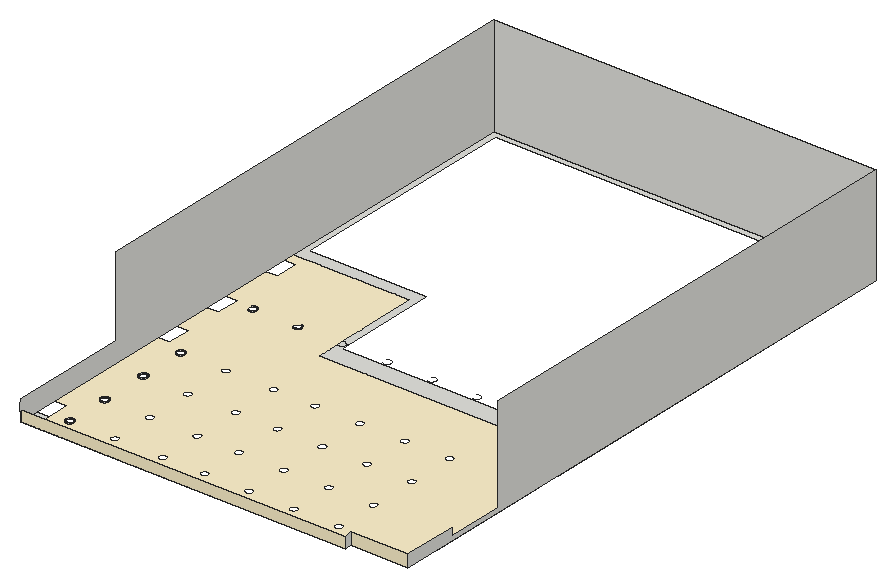
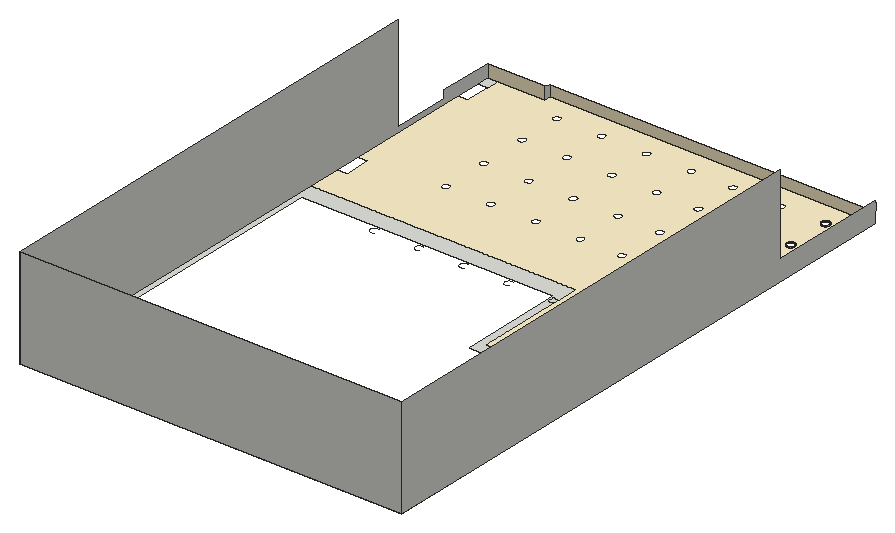
# SketchUp Ruby script. Lengths in inches.
U = 1.inch
M = Sketchup.active_model
def pt(a) = Geom::Point3d.new(a.map { |v| v * U })
def face(e, loops, mat)
  f = e.add_face(loops[0].map { |a| pt(a) })
  loops[1..].each { |l| e.add_face(l.map { |a| pt(a) }).erase! }
  f.material = f.back_material = mat if mat
  f
end
# faces: each face lists its corners as indices into pts; further lists are holes
def faces(e, pts, list, mat = nil) = list.each { |f| face(e, (f[0].is_a?(Array) ? f : [f]).map { |l| l.map { |i| pts[i] } }, mat) }
# xy, xz, yz: faces in a plane at the given z, y or x. An outline is a flat list of corners, or four numbers for a rectangle; further outlines are holes
def ring(l) = l.size == 4 ? [[l[0], l[1]], [l[2], l[1]], [l[2], l[3]], [l[0], l[3]]] : l.each_slice(2).to_a
def flat(e, list, mat, &to3) = list.each { |f| face(e, (f[0].is_a?(Array) ? f : [f]).map { |l| ring(l).map { |u, v| to3.(u, v) } }, mat) }
def xy(e, z, list, mat = nil) = flat(e, list, mat) { |x, y| [x, y, z] }
def xz(e, y, list, mat = nil) = flat(e, list, mat) { |x, z| [x, y, z] }
def yz(e, x, list, mat = nil) = flat(e, list, mat) { |y, z| [x, y, z] }
def lines(e, pts, list) = list.each { |a, b| e.add_line(pt(pts[a]), pt(pts[b])) }
# prism: a flat outline (further loops are holes) pulled along v
def prism(e, loops, v, mat = nil)
  f = face(e, loops, mat); d = Geom::Vector3d.new(v.map { |x| x * U })
  f.pushpull(f.normal.samedirection?(d) ? d.length : -d.length)
end
def box(e, o, s, mat = nil) = prism(e, [[o, [o[0] + s[0], o[1], o[2]], [o[0] + s[0], o[1] + s[1], o[2]], [o[0], o[1] + s[1], o[2]]]], [0, 0, s[2]], mat)
def at(x, y, z, deg = 0) = Geom::Transformation.translation(pt([x, y, z])) * Geom::Transformation.rotation(ORIGIN, Z_AXIS, deg.degrees)
def axes(o, x, y, z) = Geom::Transformation.new([*x, 0, *y, 0, *z, 0, *pt(o).to_a, 1])
def part(name) = M.definitions.add(name)
# library, detail: a bought-in or finely detailed component or shape, given as its bounding box
def library(name, o, s) = part(name).tap { |d| box(d.entities, o, s) }
def detail(e, o, s) = box(e.add_group.entities, o, s)
def put(e, d, t, mat = nil) = e.add_instance(d, t).tap { |i| i.material = mat if mat }
def group(e, t, mat = nil) = e.add_group.tap { |g| g.transformation = t; g.material = mat if mat }.entities
root = M.entities
M.materials.add("[Color D01]").color = [255, 242, 204]
xy(root,126,[[177.75,359.375,193.125,383.3125],[644.75,368.125,657.75,383.3125],[[324.13,645.5,324.13,673.57,324.96,672.9375,326.17,672.4375,327.46,672.27,328.76,672.4375,329.96,672.9375,331,673.73,331.79,674.77,332.29,675.97,332.46,677.27,332.29,678.5625,331.79,679.77,331,680.8,329.96,681.6,328.76,682.1,327.46,682.27,326.17,682.1,324.96,681.6,324.13,680.96,324.13,788.13,177.75,788.13,177.75,1103.3125,657.75,1103.3125,657.75,645.5],[332.57,669.6875,650.24,669.6875,650.24,1095.81,185.26,1095.81,185.26,802.9375,332.57,802.9375]],[327.46,672.27,326.17,672.4375,324.96,672.9375,324.13,673.57,324.13,680.96,324.96,681.6,326.17,682.1,327.46,682.27,328.76,682.1,329.96,681.6,331,680.8,331.79,679.77,332.29,678.5625,332.46,677.27,332.29,675.97,331.79,674.77,331,673.73,329.96,672.9375,328.76,672.4375]])
xy(root,126,[[[193.125,359.375,193.125,412.64,177.75,412.64,177.75,575.25,192.5,575.25,192.5,604.58,177.75,604.58,177.75,651.6,192.5,651.6,192.5,680.93,177.75,680.93,177.75,744.25,192.5,744.25,192.5,773.58,177.75,773.58,177.75,788.13,324.13,788.13,324.13,645.5,657.75,645.5,657.75,604.54,644.75,604.54,644.75,572.73,657.75,572.73,657.75,415.125,644.75,415.125,644.75,368.125,585.62,368.125,585.62,359.375],[271.15,500.05,272.44,500.22,273.65,500.72,274.68,501.52,275.48,502.55,275.98,503.76,276.15,505.05,275.98,506.35,275.48,507.55,274.68,508.59,273.65,509.38,272.44,509.88,271.15,510.05,269.86,509.88,268.65,509.38,267.61,508.59,266.82,507.55,266.32,506.35,266.15,505.05,266.32,503.76,266.82,502.55,267.61,501.52,268.65,500.72,269.86,500.22],[440.09,500.05,441.38,500.22,442.59,500.72,443.62,501.52,444.42,502.55,444.92,503.76,445.09,505.05,444.92,506.35,444.42,507.55,443.62,508.59,442.59,509.38,441.38,509.88,440.09,510.05,438.79,509.88,437.59,509.38,436.55,508.59,435.76,507.55,435.26,506.35,435.09,505.05,435.26,503.76,435.76,502.55,436.55,501.52,437.59,500.72,438.79,500.22],[496.4,500.05,497.69,500.22,498.9,500.72,499.93,501.52,500.73,502.55,501.23,503.76,501.4,505.05,501.23,506.35,500.73,507.55,499.93,508.59,498.9,509.38,497.69,509.88,496.4,510.05,495.11,509.88,493.9,509.38,492.86,508.59,492.07,507.55,491.57,506.35,491.4,505.05,491.57,503.76,492.07,502.55,492.86,501.52,493.9,500.72,495.11,500.22],[552.71,500.05,554.01,500.22,555.21,500.72,556.25,501.52,557.04,502.55,557.54,503.76,557.71,505.05,557.54,506.35,557.04,507.55,556.25,508.59,555.21,509.38,554.01,509.88,552.71,510.05,551.42,509.88,550.21,509.38,549.18,508.59,548.38,507.55,547.88,506.35,547.71,505.05,547.88,503.76,548.38,502.55,549.18,501.52,550.21,500.72,551.42,500.22],[271.15,439.5625,272.44,439.73,273.65,440.23,274.68,441.03,275.48,442.0625,275.98,443.27,276.15,444.5625,275.98,445.86,275.48,447.0625,274.68,448.1,273.65,448.89,272.44,449.39,271.15,449.5625,269.86,449.39,268.65,448.89,267.61,448.1,266.82,447.0625,266.32,445.86,266.15,444.5625,266.32,443.27,266.82,442.0625,267.61,441.03,268.65,440.23,269.86,439.73],[440.09,439.5625,441.38,439.73,442.59,440.23,443.62,441.03,444.42,442.0625,444.92,443.27,445.09,444.5625,444.92,445.86,444.42,447.0625,443.62,448.1,442.59,448.89,441.38,449.39,440.09,449.5625,438.79,449.39,437.59,448.89,436.55,448.1,435.76,447.0625,435.26,445.86,435.09,444.5625,435.26,443.27,435.76,442.0625,436.55,441.03,437.59,440.23,438.79,439.73],[496.4,439.5625,497.69,439.73,498.9,440.23,499.93,441.03,500.73,442.0625,501.23,443.27,501.4,444.5625,501.23,445.86,500.73,447.0625,499.93,448.1,498.9,448.89,497.69,449.39,496.4,449.5625,495.11,449.39,493.9,448.89,492.86,448.1,492.07,447.0625,491.57,445.86,491.4,444.5625,491.57,443.27,492.07,442.0625,492.86,441.03,493.9,440.23,495.11,439.73],[552.71,439.5625,554.01,439.73,555.21,440.23,556.25,441.03,557.04,442.0625,557.54,443.27,557.71,444.5625,557.54,445.86,557.04,447.0625,556.25,448.1,555.21,448.89,554.01,449.39,552.71,449.5625,551.42,449.39,550.21,448.89,549.18,448.1,548.38,447.0625,547.88,445.86,547.71,444.5625,547.88,443.27,548.38,442.0625,549.18,441.03,550.21,440.23,551.42,439.73],[271.15,672.27,272.44,672.4375,273.65,672.9375,274.68,673.73,275.48,674.77,275.98,675.97,276.15,677.27,275.98,678.5625,275.48,679.77,274.68,680.8,273.65,681.6,272.44,682.1,271.15,682.27,269.86,682.1,268.65,681.6,267.61,680.8,266.82,679.77,266.32,678.5625,266.15,677.27,266.32,675.97,266.82,674.77,267.61,673.73,268.65,672.9375,269.86,672.4375],[271.15,559.33,272.44,559.5,273.65,560,274.68,560.79,275.48,561.83,275.98,563.03,276.15,564.33,275.98,565.62,275.48,566.83,274.68,567.86,273.65,568.66,272.44,569.16,271.15,569.33,269.86,569.16,268.65,568.66,267.61,567.86,266.82,566.83,266.32,565.62,266.15,564.33,266.32,563.03,266.82,561.83,267.61,560.79,268.65,560,269.86,559.5],[440.09,559.33,441.38,559.5,442.59,560,443.62,560.79,444.42,561.83,444.92,563.03,445.09,564.33,444.92,565.62,444.42,566.83,443.62,567.86,442.59,568.66,441.38,569.16,440.09,569.33,438.79,569.16,437.59,568.66,436.55,567.86,435.76,566.83,435.26,565.62,435.09,564.33,435.26,563.03,435.76,561.83,436.55,560.79,437.59,560,438.79,559.5],[496.4,559.33,497.69,559.5,498.9,560,499.93,560.79,500.73,561.83,501.23,563.03,501.4,564.33,501.23,565.62,500.73,566.83,499.93,567.86,498.9,568.66,497.69,569.16,496.4,569.33,495.11,569.16,493.9,568.66,492.86,567.86,492.07,566.83,491.57,565.62,491.4,564.33,491.57,563.03,492.07,561.83,492.86,560.79,493.9,560,495.11,559.5],[552.71,559.33,554.01,559.5,555.21,560,556.25,560.79,557.04,561.83,557.54,563.03,557.71,564.33,557.54,565.62,557.04,566.83,556.25,567.86,555.21,568.66,554.01,569.16,552.71,569.33,551.42,569.16,550.21,568.66,549.18,567.86,548.38,566.83,547.88,565.62,547.71,564.33,547.88,563.03,548.38,561.83,549.18,560.79,550.21,560,551.42,559.5],[271.15,385.12,272.44,385.29,273.65,385.79,274.68,386.58,275.48,387.62,275.98,388.83,276.15,390.12,275.98,391.41,275.48,392.62,274.68,393.66,273.65,394.45,272.44,394.95,271.15,395.12,269.86,394.95,268.65,394.45,267.61,393.66,266.82,392.62,266.32,391.41,266.15,390.12,266.32,388.83,266.82,387.62,267.61,386.58,268.65,385.79,269.86,385.29],[440.09,385.12,441.38,385.29,442.59,385.79,443.62,386.58,444.42,387.62,444.92,388.83,445.09,390.12,444.92,391.41,444.42,392.62,443.62,393.66,442.59,394.45,441.38,394.95,440.09,395.12,438.79,394.95,437.59,394.45,436.55,393.66,435.76,392.62,435.26,391.41,435.09,390.12,435.26,388.83,435.76,387.62,436.55,386.58,437.59,385.79,438.79,385.29],[496.4,385.12,497.69,385.29,498.9,385.79,499.93,386.58,500.73,387.62,501.23,388.83,501.4,390.12,501.23,391.41,500.73,392.62,499.93,393.66,498.9,394.45,497.69,394.95,496.4,395.12,495.11,394.95,493.9,394.45,492.86,393.66,492.07,392.62,491.57,391.41,491.4,390.12,491.57,388.83,492.07,387.62,492.86,386.58,493.9,385.79,495.11,385.29],[552.71,385.12,554.01,385.29,555.21,385.79,556.25,386.58,557.04,387.62,557.54,388.83,557.71,390.12,557.54,391.41,557.04,392.62,556.25,393.66,555.21,394.45,554.01,394.95,552.71,395.12,551.42,394.95,550.21,394.45,549.18,393.66,548.38,392.62,547.88,391.41,547.71,390.12,547.88,388.83,548.38,387.62,549.18,386.58,550.21,385.79,551.42,385.29],[214.84,672.27,216.13,672.4375,217.34,672.9375,218.37,673.73,219.17,674.77,219.67,675.97,219.84,677.27,219.67,678.5625,219.17,679.77,218.37,680.8,217.34,681.6,216.13,682.1,214.84,682.27,213.54,682.1,212.34,681.6,211.3,680.8,210.51,679.77,210.01,678.5625,209.84,677.27,210.01,675.97,210.51,674.77,211.3,673.73,212.34,672.9375,213.54,672.4375],[214.84,439.5625,216.13,439.73,217.34,440.23,218.37,441.03,219.17,442.0625,219.67,443.27,219.84,444.5625,219.67,445.86,219.17,447.0625,218.37,448.1,217.34,448.89,216.13,449.39,214.84,449.5625,213.54,449.39,212.34,448.89,211.3,448.1,210.51,447.0625,210.01,445.86,209.84,444.5625,210.01,443.27,210.51,442.0625,211.3,441.03,212.34,440.23,213.54,439.73],[214.84,500.05,216.13,500.22,217.34,500.72,218.37,501.52,219.17,502.55,219.67,503.76,219.84,505.05,219.67,506.35,219.17,507.55,218.37,508.59,217.34,509.38,216.13,509.88,214.84,510.05,213.54,509.88,212.34,509.38,211.3,508.59,210.51,507.55,210.01,506.35,209.84,505.05,210.01,503.76,210.51,502.55,211.3,501.52,212.34,500.72,213.54,500.22],[214.84,559.33,216.13,559.5,217.34,560,218.37,560.79,219.17,561.83,219.67,563.03,219.84,564.33,219.67,565.62,219.17,566.83,218.37,567.86,217.34,568.66,216.13,569.16,214.84,569.33,213.54,569.16,212.34,568.66,211.3,567.86,210.51,566.83,210.01,565.62,209.84,564.33,210.01,563.03,210.51,561.83,211.3,560.79,212.34,560,213.54,559.5],[214.84,385.12,216.13,385.29,217.34,385.79,218.37,386.58,219.17,387.62,219.67,388.83,219.84,390.12,219.67,391.41,219.17,392.62,218.37,393.66,217.34,394.45,216.13,394.95,214.84,395.12,213.54,394.95,212.34,394.45,211.3,393.66,210.51,392.62,210.01,391.41,209.84,390.12,210.01,388.83,210.51,387.62,211.3,386.58,212.34,385.79,213.54,385.29],[331.21,439.5625,332.51,439.73,333.71,440.23,334.75,441.03,335.54,442.0625,336.04,443.27,336.21,444.5625,336.04,445.86,335.54,447.0625,334.75,448.1,333.71,448.89,332.51,449.39,331.21,449.5625,329.92,449.39,328.71,448.89,327.68,448.1,326.88,447.0625,326.38,445.86,326.21,444.5625,326.38,443.27,326.88,442.0625,327.68,441.03,328.71,440.23,329.92,439.73],[383.77,439.5625,385.07,439.73,386.27,440.23,387.31,441.03,388.1,442.0625,388.6,443.27,388.77,444.5625,388.6,445.86,388.1,447.0625,387.31,448.1,386.27,448.89,385.07,449.39,383.77,449.5625,382.48,449.39,381.27,448.89,380.24,448.1,379.44,447.0625,378.94,445.86,378.77,444.5625,378.94,443.27,379.44,442.0625,380.24,441.03,381.27,440.23,382.48,439.73],[383.77,500.05,385.07,500.22,386.27,500.72,387.31,501.52,388.1,502.55,388.6,503.76,388.77,505.05,388.6,506.35,388.1,507.55,387.31,508.59,386.27,509.38,385.07,509.88,383.77,510.05,382.48,509.88,381.27,509.38,380.24,508.59,379.44,507.55,378.94,506.35,378.77,505.05,378.94,503.76,379.44,502.55,380.24,501.52,381.27,500.72,382.48,500.22],[331.21,500.05,332.51,500.22,333.71,500.72,334.75,501.52,335.54,502.55,336.04,503.76,336.21,505.05,336.04,506.35,335.54,507.55,334.75,508.59,333.71,509.38,332.51,509.88,331.21,510.05,329.92,509.88,328.71,509.38,327.68,508.59,326.88,507.55,326.38,506.35,326.21,505.05,326.38,503.76,326.88,502.55,327.68,501.52,328.71,500.72,329.92,500.22],[383.77,559.33,385.07,559.5,386.27,560,387.31,560.79,388.1,561.83,388.6,563.03,388.77,564.33,388.6,565.62,388.1,566.83,387.31,567.86,386.27,568.66,385.07,569.16,383.77,569.33,382.48,569.16,381.27,568.66,380.24,567.86,379.44,566.83,378.94,565.62,378.77,564.33,378.94,563.03,379.44,561.83,380.24,560.79,381.27,560,382.48,559.5],[331.21,559.33,332.51,559.5,333.71,560,334.75,560.79,335.54,561.83,336.04,563.03,336.21,564.33,336.04,565.62,335.54,566.83,334.75,567.86,333.71,568.66,332.51,569.16,331.21,569.33,329.92,569.16,328.71,568.66,327.68,567.86,326.88,566.83,326.38,565.62,326.21,564.33,326.38,563.03,326.88,561.83,327.68,560.79,328.71,560,329.92,559.5],[383.77,385.12,385.07,385.29,386.27,385.79,387.31,386.58,388.1,387.62,388.6,388.83,388.77,390.12,388.6,391.41,388.1,392.62,387.31,393.66,386.27,394.45,385.07,394.95,383.77,395.12,382.48,394.95,381.27,394.45,380.24,393.66,379.44,392.62,378.94,391.41,378.77,390.12,378.94,388.83,379.44,387.62,380.24,386.58,381.27,385.79,382.48,385.29],[331.21,385.12,332.51,385.29,333.71,385.79,334.75,386.58,335.54,387.62,336.04,388.83,336.21,390.12,336.04,391.41,335.54,392.62,334.75,393.66,333.71,394.45,332.51,394.95,331.21,395.12,329.92,394.95,328.71,394.45,327.68,393.66,326.88,392.62,326.38,391.41,326.21,390.12,326.38,388.83,326.88,387.62,327.68,386.58,328.71,385.79,329.92,385.29]]],"[Color D01]")
xz(root,359.375,[[177.75,126,585.62,139.1]],"[Color D01]")
xz(root,368.125,[[585.62,126,657.75,141.4375]],"[Color D01]")
xz(root,1103.3125,[[177.75,126,657.75,252]])
yz(root,177.75,[[359.375,126,359.375,139.1,357.25,139.1,357.25,148.36,359.375,148.36,359.375,151.5,508.37,151.5,508.37,252,1103.3125,252,1103.3125,126]])
yz(root,585.62,[[359.375,126,368.125,126,368.125,141.4375,359.375,139.1]])
yz(root,657.75,[[368.125,126,1103.3125,126,1103.3125,252,508.37,252,508.37,132,436.28,132,436.28,141.4375,368.125,141.4375]])
p = [[214.84,385.12,126],[213.54,385.29,126],[213.54,385.29,126.875],[214.84,385.12,126.875],[216.13,385.29,126],[216.13,385.29,126.875],
  [212.34,385.79,126],[212.34,385.79,126.875],[217.34,385.79,126],[217.34,385.79,126.875],[211.3,386.58,126],[211.3,386.58,126.875],
  [218.37,386.58,126],[218.37,386.58,126.875],[210.51,387.62,126],[210.51,387.62,126.875],[219.17,387.62,126],[219.17,387.62,126.875],
  [210.01,388.83,126],[210.01,388.83,126.875],[219.67,388.83,126],[219.67,388.83,126.875],[209.84,390.12,126],[209.84,390.12,126.875],
  [219.84,390.12,126],[219.84,390.12,126.875],[210.01,391.41,126],[210.01,391.41,126.875],[219.67,391.41,126],[219.67,391.41,126.875],
  [210.51,392.62,126],[210.51,392.62,126.875],[219.17,392.62,126],[219.17,392.62,126.875],[211.3,393.66,126],[211.3,393.66,126.875],
  [218.37,393.66,126],[218.37,393.66,126.875],[212.34,394.45,126],[212.34,394.45,126.875],[217.34,394.45,126],[217.34,394.45,126.875],
  [213.54,394.95,126],[213.54,394.95,126.875],[216.13,394.95,126],[216.13,394.95,126.875],[214.84,395.12,126],[214.84,395.12,126.875],
  [214.84,439.5625,126],[213.54,439.73,126],[213.54,439.73,126.875],[214.84,439.5625,126.875],[216.13,439.73,126],[216.13,439.73,126.875],
  [212.34,440.23,126],[212.34,440.23,126.875],[217.34,440.23,126],[217.34,440.23,126.875],[211.3,441.03,126],[211.3,441.03,126.875],
  [218.37,441.03,126],[218.37,441.03,126.875],[210.51,442.0625,126],[210.51,442.0625,126.875],[219.17,442.0625,126],[219.17,442.0625,126.875],
  [210.01,443.27,126],[210.01,443.27,126.875],[219.67,443.27,126],[219.67,443.27,126.875],[209.84,444.5625,126],[209.84,444.5625,126.875],
  [219.84,444.5625,126],[219.84,444.5625,126.875],[210.01,445.86,126],[210.01,445.86,126.875],[219.67,445.86,126],[219.67,445.86,126.875],
  [210.51,447.0625,126],[210.51,447.0625,126.875],[219.17,447.0625,126],[219.17,447.0625,126.875],[211.3,448.1,126],[211.3,448.1,126.875],
  [218.37,448.1,126],[218.37,448.1,126.875],[212.34,448.89,126],[212.34,448.89,126.875],[217.34,448.89,126],[217.34,448.89,126.875],
  [213.54,449.39,126],[213.54,449.39,126.875],[216.13,449.39,126],[216.13,449.39,126.875],[214.84,449.5625,126],[214.84,449.5625,126.875],
  [214.84,500.05,126],[213.54,500.22,126],[213.54,500.22,126.875],[214.84,500.05,126.875],[216.13,500.22,126],[216.13,500.22,126.875],
  [212.34,500.72,126],[212.34,500.72,126.875],[217.34,500.72,126],[217.34,500.72,126.875],[211.3,501.52,126],[211.3,501.52,126.875],
  [218.37,501.52,126],[218.37,501.52,126.875],[210.51,502.55,126],[210.51,502.55,126.875],[219.17,502.55,126],[219.17,502.55,126.875],
  [210.01,503.76,126],[210.01,503.76,126.875],[219.67,503.76,126],[219.67,503.76,126.875],[209.84,505.05,126],[209.84,505.05,126.875],
  [219.84,505.05,126],[219.84,505.05,126.875],[210.01,506.35,126],[210.01,506.35,126.875],[219.67,506.35,126],[219.67,506.35,126.875],
  [210.51,507.55,126],[210.51,507.55,126.875],[219.17,507.55,126],[219.17,507.55,126.875],[211.3,508.59,126],[211.3,508.59,126.875],
  [218.37,508.59,126],[218.37,508.59,126.875],[212.34,509.38,126],[212.34,509.38,126.875],[217.34,509.38,126],[217.34,509.38,126.875],
  [213.54,509.88,126],[213.54,509.88,126.875],[216.13,509.88,126],[216.13,509.88,126.875],[214.84,510.05,126],[214.84,510.05,126.875],
  [214.84,559.33,126],[213.54,559.5,126],[213.54,559.5,126.875],[214.84,559.33,126.875],[216.13,559.5,126],[216.13,559.5,126.875],
  [212.34,560,126],[212.34,560,126.875],[217.34,560,126],[217.34,560,126.875],[211.3,560.79,126],[211.3,560.79,126.875],
  [218.37,560.79,126],[218.37,560.79,126.875],[210.51,561.83,126],[210.51,561.83,126.875],[219.17,561.83,126],[219.17,561.83,126.875],
  [210.01,563.03,126],[210.01,563.03,126.875],[219.67,563.03,126],[219.67,563.03,126.875],[209.84,564.33,126],[209.84,564.33,126.875],
  [219.84,564.33,126],[219.84,564.33,126.875],[210.01,565.62,126],[210.01,565.62,126.875],[219.67,565.62,126],[219.67,565.62,126.875],
  [210.51,566.83,126],[210.51,566.83,126.875],[219.17,566.83,126],[219.17,566.83,126.875],[211.3,567.86,126],[211.3,567.86,126.875],
  [218.37,567.86,126],[218.37,567.86,126.875],[212.34,568.66,126],[212.34,568.66,126.875],[217.34,568.66,126],[217.34,568.66,126.875],
  [213.54,569.16,126],[213.54,569.16,126.875],[216.13,569.16,126],[216.13,569.16,126.875],[214.84,569.33,126],[214.84,569.33,126.875],
  [214.84,672.27,126],[213.54,672.4375,126],[213.54,672.4375,126.875],[214.84,672.27,126.875],[216.13,672.4375,126],[216.13,672.4375,126.875],
  [271.15,672.27,126],[269.86,672.4375,126],[269.86,672.4375,126.875],[271.15,672.27,126.875],[272.44,672.4375,126],[272.44,672.4375,126.875],
  [212.34,672.9375,126],[212.34,672.9375,126.875],[217.34,672.9375,126],[217.34,672.9375,126.875],[268.65,672.9375,126],[268.65,672.9375,126.875],
  [273.65,672.9375,126],[273.65,672.9375,126.875],[218.37,673.73,126],[218.37,673.73,126.875],[274.68,673.73,126],[274.68,673.73,126.875],
  [219.17,674.77,126],[219.17,674.77,126.875],[275.48,674.77,126],[275.48,674.77,126.875],[219.67,675.97,126],[219.67,675.97,126.875],
  [275.98,675.97,126],[275.98,675.97,126.875],[219.84,677.27,126],[219.84,677.27,126.875],[276.15,677.27,126],[276.15,677.27,126.875],
  [219.67,678.5625,126],[219.67,678.5625,126.875],[275.98,678.5625,126],[275.98,678.5625,126.875],[219.17,679.77,126],[219.17,679.77,126.875],
  [275.48,679.77,126],[275.48,679.77,126.875],[218.37,680.8,126],[218.37,680.8,126.875],[274.68,680.8,126],[274.68,680.8,126.875],
  [211.3,680.8,126],[212.34,681.6,126],[212.34,681.6,126.875],[211.3,680.8,126.875],[217.34,681.6,126],[217.34,681.6,126.875],
  [273.65,681.6,126],[273.65,681.6,126.875],[213.54,682.1,126],[213.54,682.1,126.875],[216.13,682.1,126],[216.13,682.1,126.875],
  [272.44,682.1,126],[272.44,682.1,126.875],[214.84,682.27,126],[214.84,682.27,126.875],[388.1,679.77,126],[387.31,680.8,126],
  [388.77,677.27,126],[388.6,678.5625,126],[386.27,681.6,126],[385.07,682.1,126],[383.77,682.27,126],[382.48,682.1,126],
  [381.27,681.6,126],[380.24,680.8,126],[381.27,672.9375,126],[382.48,672.4375,126],[383.77,672.27,126],[385.07,672.4375,126],
  [386.27,672.9375,126],[387.31,673.73,126],[388.1,674.77,126],[388.6,675.97,126],[444.42,679.77,126],[443.62,680.8,126],
  [445.09,677.27,126],[444.92,678.5625,126],[442.59,681.6,126],[441.38,682.1,126],[440.09,682.27,126],[438.79,682.1,126],
  [437.59,681.6,126],[436.55,680.8,126],[437.59,672.9375,126],[438.79,672.4375,126],[440.09,672.27,126],[441.38,672.4375,126],
  [442.59,672.9375,126],[443.62,673.73,126],[444.42,674.77,126],[444.92,675.97,126],[500.73,679.77,126],[499.93,680.8,126],
  [501.4,677.27,126],[501.23,678.5625,126],[498.9,681.6,126],[497.69,682.1,126],[496.4,682.27,126],[495.11,682.1,126],
  [493.9,681.6,126],[492.86,680.8,126],[493.9,672.9375,126],[495.11,672.4375,126],[496.4,672.27,126],[497.69,672.4375,126],
  [498.9,672.9375,126],[499.93,673.73,126],[500.73,674.77,126],[501.23,675.97,126],[557.04,679.77,126],[556.25,680.8,126],
  [557.71,677.27,126],[557.54,678.5625,126],[555.21,681.6,126],[554.01,682.1,126],[552.71,682.27,126],[551.42,682.1,126],
  [550.21,681.6,126],[549.18,680.8,126],[550.21,672.9375,126],[551.42,672.4375,126],[552.71,672.27,126],[554.01,672.4375,126],
  [555.21,672.9375,126],[556.25,673.73,126],[557.04,674.77,126],[557.54,675.97,126]]
faces(root,p,[[0,1,2,3],[4,0,3,5],[1,6,7,2],[8,4,5,9],[6,10,11,7],[12,8,9,13],[10,14,15,11],[16,12,13,17],
  [14,18,19,15],[20,16,17,21],[18,22,23,19],[24,20,21,25],[22,26,27,23],[28,24,25,29],[26,30,31,27],[32,28,29,33],
  [30,34,35,31],[36,32,33,37],[34,38,39,35],[40,36,37,41],[38,42,43,39],[44,40,41,45],[42,46,47,43],[46,44,45,47],
  [48,49,50,51],[52,48,51,53],[49,54,55,50],[56,52,53,57],[54,58,59,55],[60,56,57,61],[58,62,63,59],[64,60,61,65],
  [62,66,67,63],[68,64,65,69],[66,70,71,67],[72,68,69,73],[70,74,75,71],[76,72,73,77],[74,78,79,75],[80,76,77,81],
  [78,82,83,79],[84,80,81,85],[82,86,87,83],[88,84,85,89],[86,90,91,87],[92,88,89,93],[90,94,95,91],[94,92,93,95],
  [96,97,98,99],[100,96,99,101],[97,102,103,98],[104,100,101,105],[102,106,107,103],[108,104,105,109],[106,110,111,107],[112,108,109,113],
  [110,114,115,111],[116,112,113,117],[114,118,119,115],[120,116,117,121],[118,122,123,119],[124,120,121,125],[122,126,127,123],[128,124,125,129],
  [126,130,131,127],[132,128,129,133],[130,134,135,131],[136,132,133,137],[134,138,139,135],[140,136,137,141],[138,142,143,139],[142,140,141,143],
  [144,145,146,147],[148,144,147,149],[145,150,151,146],[152,148,149,153],[150,154,155,151],[156,152,153,157],[154,158,159,155],[160,156,157,161],
  [158,162,163,159],[164,160,161,165],[162,166,167,163],[168,164,165,169],[166,170,171,167],[172,168,169,173],[170,174,175,171],[176,172,173,177],
  [174,178,179,175],[180,176,177,181],[178,182,183,179],[184,180,181,185],[182,186,187,183],[188,184,185,189],[186,190,191,187],[190,188,189,191],
  [192,193,194,195],[196,192,195,197],[198,199,200,201],[202,198,201,203],[193,204,205,194],[206,196,197,207],[199,208,209,200],[210,202,203,211],
  [212,206,207,213],[214,210,211,215],[216,212,213,217],[218,214,215,219],[220,216,217,221],[222,218,219,223],[224,220,221,225],[226,222,223,227],
  [228,224,225,229],[230,226,227,231],[232,228,229,233],[234,230,231,235],[236,232,233,237],[238,234,235,239],[240,241,242,243],[244,236,237,245],
  [246,238,239,247],[241,248,249,242],[250,244,245,251],[252,246,247,253],[248,254,255,249],[254,250,251,255]])
lines(root,p,[[256,257],[258,259],[259,256],[257,260],[260,261],[261,262],[262,263],[263,264],[264,265],[266,267],[267,268],[268,269],
  [269,270],[270,271],[271,272],[272,273],[273,258],[274,275],[276,277],[277,274],[275,278],[278,279],[279,280],[280,281],
  [281,282],[282,283],[284,285],[285,286],[286,287],[287,288],[288,289],[289,290],[290,291],[291,276],[292,293],[294,295],
  [295,292],[293,296],[296,297],[297,298],[298,299],[299,300],[300,301],[302,303],[303,304],[304,305],[305,306],[306,307],
  [307,308],[308,309],[309,294],[310,311],[312,313],[313,310],[311,314],[314,315],[315,316],[316,317],[317,318],[318,319],
  [320,321],[321,322],[322,323],[323,324],[324,325],[325,326],[326,327],[327,312]])
